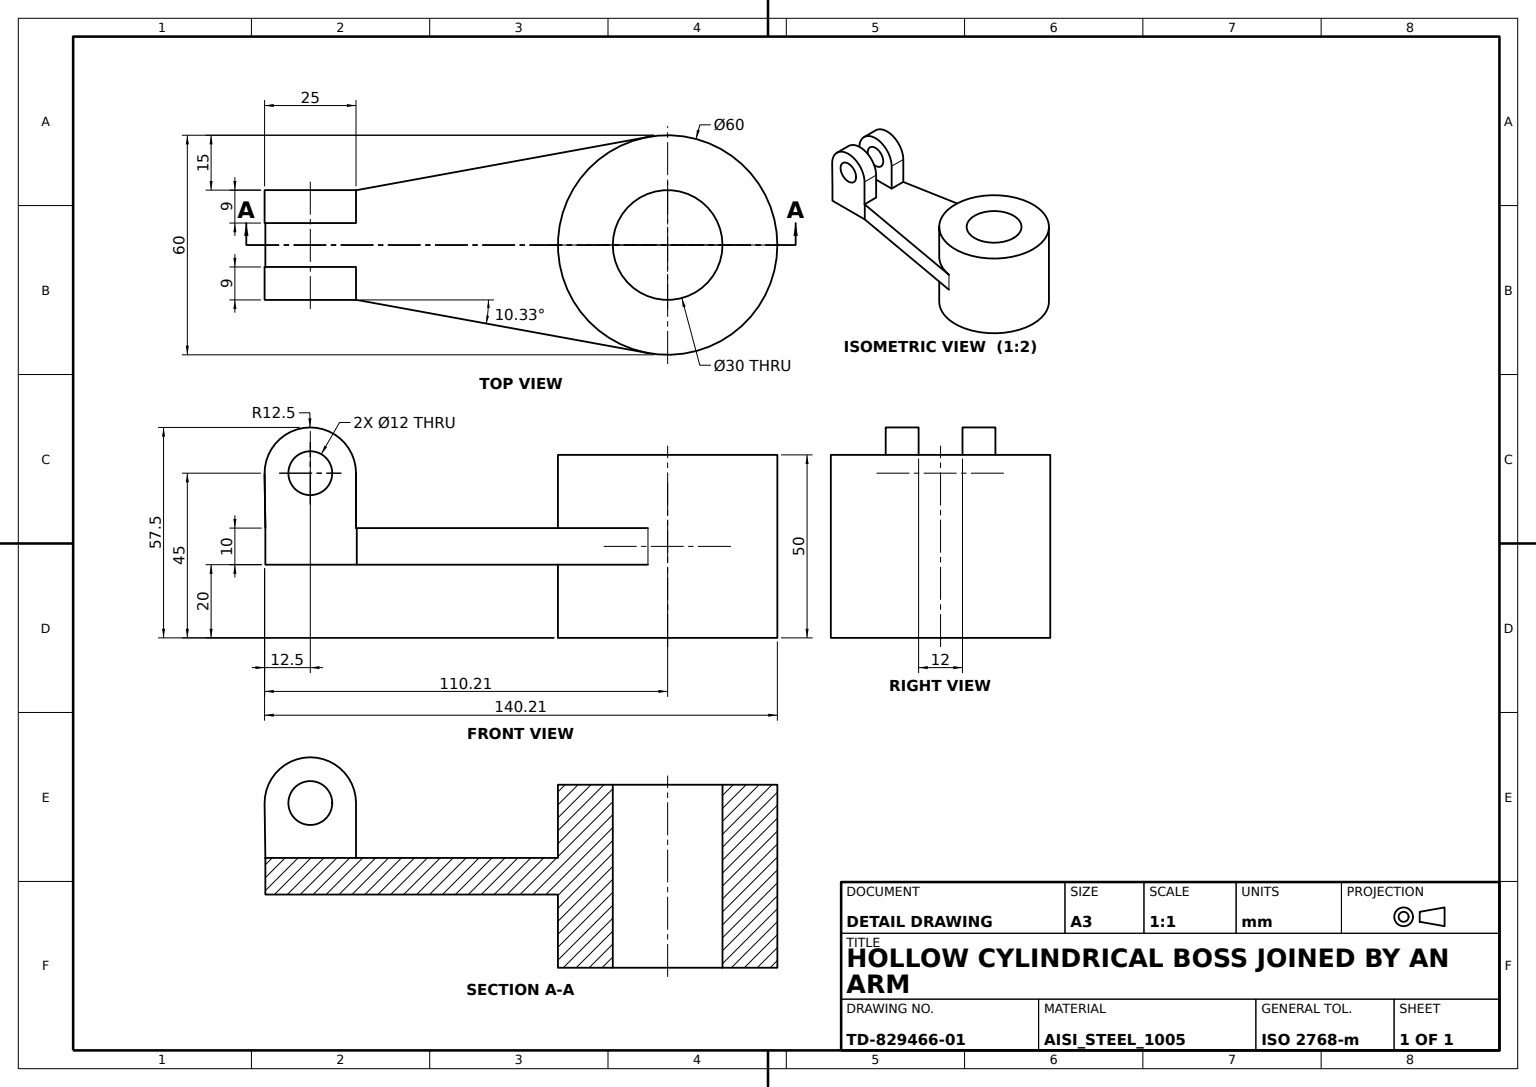
ISO-10303-21;
HEADER;
FILE_DESCRIPTION((''),'2;1');
FILE_NAME('','',(''),(''),'','','');
FILE_SCHEMA(('AUTOMOTIVE_DESIGN'));
ENDSEC;
DATA;
#1=APPLICATION_CONTEXT('');
#2=PRODUCT_CONTEXT('',#1,'mechanical');
#3=PRODUCT('','','',(#2));
#4=PRODUCT_DEFINITION_FORMATION('','',#3);
#5=PRODUCT_DEFINITION_CONTEXT('',#1,'design');
#6=PRODUCT_DEFINITION('','',#4,#5);
#7=PRODUCT_DEFINITION_SHAPE('','',#6);
#8=(LENGTH_UNIT()NAMED_UNIT(*)SI_UNIT(.MILLI.,.METRE.));
#9=(NAMED_UNIT(*)PLANE_ANGLE_UNIT()SI_UNIT($,.RADIAN.));
#10=(NAMED_UNIT(*)SI_UNIT($,.STERADIAN.)SOLID_ANGLE_UNIT());
#11=UNCERTAINTY_MEASURE_WITH_UNIT(LENGTH_MEASURE(0.005),#8,'distance_accuracy_value','');
#12=(GEOMETRIC_REPRESENTATION_CONTEXT(3)GLOBAL_UNCERTAINTY_ASSIGNED_CONTEXT((#11))GLOBAL_UNIT_ASSIGNED_CONTEXT((#8,#9,#10))REPRESENTATION_CONTEXT('',''));
#13=CARTESIAN_POINT('',(-85.210715,-6.,20.));
#14=VERTEX_POINT('',#13);
#15=CARTESIAN_POINT('',(-85.210715,-6.,5.));
#16=VERTEX_POINT('',#15);
#17=DIRECTION('',(0.,0.,-1.));
#18=VECTOR('',#17,1000.);
#19=LINE('',#13,#18);
#20=EDGE_CURVE('',#14,#16,#19,.T.);
#21=ORIENTED_EDGE('',*,*,#20,.F.);
#22=CARTESIAN_POINT('',(-85.210715,-15.,20.));
#23=VERTEX_POINT('',#22);
#24=DIRECTION('',(0.,-1.,0.));
#25=VECTOR('',#24,1000.);
#26=LINE('',#13,#25);
#27=EDGE_CURVE('',#14,#23,#26,.T.);
#28=ORIENTED_EDGE('',*,*,#27,.T.);
#29=CARTESIAN_POINT('',(-85.210715,-15.,5.));
#30=VERTEX_POINT('',#29);
#31=LINE('',#22,#18);
#32=EDGE_CURVE('',#23,#30,#31,.T.);
#33=ORIENTED_EDGE('',*,*,#32,.T.);
#34=LINE('',#15,#25);
#35=EDGE_CURVE('',#16,#30,#34,.T.);
#36=ORIENTED_EDGE('',*,*,#35,.F.);
#37=EDGE_LOOP('',(#21,#28,#33,#36));
#38=FACE_BOUND('',#37,.T.);
#39=DIRECTION('',(-1.,0.,0.));
#40=DIRECTION('',(0.,0.,1.));
#41=AXIS2_PLACEMENT_3D('',#13,#39,#40);
#42=PLANE('',#41);
#43=ADVANCED_FACE('',(#38),#42,.F.);
#44=CARTESIAN_POINT('',(-85.,15.,5.));
#45=VERTEX_POINT('',#44);
#46=CARTESIAN_POINT('',(-85.210715,15.,5.));
#47=VERTEX_POINT('',#46);
#48=VECTOR('',#39,1000.);
#49=LINE('',#44,#48);
#50=EDGE_CURVE('',#45,#47,#49,.T.);
#51=ORIENTED_EDGE('',*,*,#50,.T.);
#52=CARTESIAN_POINT('',(-85.210715,6.,5.));
#53=VERTEX_POINT('',#52);
#54=DIRECTION('',(0.,1.,0.));
#55=VECTOR('',#54,1000.);
#56=LINE('',#52,#55);
#57=EDGE_CURVE('',#53,#47,#56,.T.);
#58=ORIENTED_EDGE('',*,*,#57,.F.);
#59=CARTESIAN_POINT('',(-110.,6.,5.));
#60=VERTEX_POINT('',#59);
#61=LINE('',#52,#48);
#62=EDGE_CURVE('',#53,#60,#61,.T.);
#63=ORIENTED_EDGE('',*,*,#62,.T.);
#64=CARTESIAN_POINT('',(-110.,-6.,5.));
#65=VERTEX_POINT('',#64);
#66=CARTESIAN_POINT('',(-110.,15.,5.));
#67=LINE('',#66,#25);
#68=EDGE_CURVE('',#60,#65,#67,.T.);
#69=ORIENTED_EDGE('',*,*,#68,.T.);
#70=LINE('',#15,#48);
#71=EDGE_CURVE('',#16,#65,#70,.T.);
#72=ORIENTED_EDGE('',*,*,#71,.F.);
#73=ORIENTED_EDGE('',*,*,#35,.T.);
#74=CARTESIAN_POINT('',(-85.,-15.,5.));
#75=VERTEX_POINT('',#74);
#76=CARTESIAN_POINT('',(-110.,-15.,5.));
#77=DIRECTION('',(1.,0.,0.));
#78=VECTOR('',#77,1000.);
#79=LINE('',#76,#78);
#80=EDGE_CURVE('',#30,#75,#79,.T.);
#81=ORIENTED_EDGE('',*,*,#80,.T.);
#82=CARTESIAN_POINT('',(-5.379942,-29.513662,5.));
#83=VERTEX_POINT('',#82);
#84=DIRECTION('',(0.983788721,-0.179331402,0.));
#85=VECTOR('',#84,1000.);
#86=LINE('',#74,#85);
#87=EDGE_CURVE('',#75,#83,#86,.T.);
#88=ORIENTED_EDGE('',*,*,#87,.T.);
#89=CARTESIAN_POINT('',(-5.379942,29.513662,5.));
#90=VERTEX_POINT('',#89);
#91=CARTESIAN_POINT('',(0.,0.,5.));
#92=AXIS2_PLACEMENT_3D('',#91,#17,#77);
#93=CIRCLE('',#92,30.);
#94=EDGE_CURVE('',#83,#90,#93,.T.);
#95=ORIENTED_EDGE('',*,*,#94,.T.);
#96=DIRECTION('',(-0.983788721,-0.179331402,0.));
#97=VECTOR('',#96,1000.);
#98=LINE('',#89,#97);
#99=EDGE_CURVE('',#90,#45,#98,.T.);
#100=ORIENTED_EDGE('',*,*,#99,.T.);
#101=EDGE_LOOP('',(#51,#58,#63,#69,#72,#73,#81,#88,#95,#100));
#102=FACE_BOUND('',#101,.T.);
#103=AXIS2_PLACEMENT_3D('',#91,#17,#39);
#104=PLANE('',#103);
#105=ADVANCED_FACE('',(#102),#104,.F.);
#106=CARTESIAN_POINT('',(-110.209467,-6.,19.823382));
#107=VERTEX_POINT('',#106);
#108=DIRECTION('',(-0.014129422,0.,0.999900175));
#109=VECTOR('',#108,1000.);
#110=LINE('',#64,#109);
#111=EDGE_CURVE('',#65,#107,#110,.T.);
#112=ORIENTED_EDGE('',*,*,#111,.F.);
#113=VERTEX_POINT('',#76);
#114=LINE('',#64,#25);
#115=EDGE_CURVE('',#65,#113,#114,.T.);
#116=ORIENTED_EDGE('',*,*,#115,.T.);
#117=CARTESIAN_POINT('',(-110.209467,-15.,19.823382));
#118=VERTEX_POINT('',#117);
#119=LINE('',#76,#109);
#120=EDGE_CURVE('',#113,#118,#119,.T.);
#121=ORIENTED_EDGE('',*,*,#120,.T.);
#122=LINE('',#106,#25);
#123=EDGE_CURVE('',#107,#118,#122,.T.);
#124=ORIENTED_EDGE('',*,*,#123,.F.);
#125=EDGE_LOOP('',(#112,#116,#121,#124));
#126=FACE_BOUND('',#125,.T.);
#127=DIRECTION('',(0.999900175,0.,0.014129422));
#128=DIRECTION('',(0.014129422,0.,-0.999900175));
#129=AXIS2_PLACEMENT_3D('',#64,#127,#128);
#130=PLANE('',#129);
#131=ADVANCED_FACE('',(#126),#130,.F.);
#132=CARTESIAN_POINT('',(15.,0.,25.));
#133=VERTEX_POINT('',#132);
#134=CARTESIAN_POINT('',(0.,0.,25.));
#135=AXIS2_PLACEMENT_3D('',#134,#40,#77);
#136=CIRCLE('',#135,15.);
#137=EDGE_CURVE('',#133,#133,#136,.T.);
#138=ORIENTED_EDGE('',*,*,#137,.T.);
#139=EDGE_LOOP('',(#138));
#140=FACE_BOUND('',#139,.T.);
#141=CARTESIAN_POINT('',(15.,0.,-25.));
#142=VERTEX_POINT('',#141);
#143=CARTESIAN_POINT('',(0.,0.,-25.));
#144=AXIS2_PLACEMENT_3D('',#143,#40,#77);
#145=CIRCLE('',#144,15.);
#146=EDGE_CURVE('',#142,#142,#145,.T.);
#147=ORIENTED_EDGE('',*,*,#146,.F.);
#148=EDGE_LOOP('',(#147));
#149=FACE_BOUND('',#148,.T.);
#150=AXIS2_PLACEMENT_3D('',#134,#17,#39);
#151=CYLINDRICAL_SURFACE('',#150,15.);
#152=ADVANCED_FACE('',(#140,#149),#151,.F.);
#153=VERTEX_POINT('',#66);
#154=CARTESIAN_POINT('',(-110.,15.,-5.));
#155=VERTEX_POINT('',#154);
#156=LINE('',#66,#18);
#157=EDGE_CURVE('',#153,#155,#156,.T.);
#158=ORIENTED_EDGE('',*,*,#157,.T.);
#159=CARTESIAN_POINT('',(-110.,-15.,-5.));
#160=VERTEX_POINT('',#159);
#161=LINE('',#154,#25);
#162=EDGE_CURVE('',#155,#160,#161,.T.);
#163=ORIENTED_EDGE('',*,*,#162,.T.);
#164=LINE('',#76,#18);
#165=EDGE_CURVE('',#113,#160,#164,.T.);
#166=ORIENTED_EDGE('',*,*,#165,.F.);
#167=ORIENTED_EDGE('',*,*,#115,.F.);
#168=ORIENTED_EDGE('',*,*,#68,.F.);
#169=EDGE_CURVE('',#153,#60,#67,.T.);
#170=ORIENTED_EDGE('',*,*,#169,.F.);
#171=EDGE_LOOP('',(#158,#163,#166,#167,#168,#170));
#172=FACE_BOUND('',#171,.T.);
#173=AXIS2_PLACEMENT_3D('',#66,#77,#17);
#174=PLANE('',#173);
#175=ADVANCED_FACE('',(#172),#174,.F.);
#176=CARTESIAN_POINT('',(-110.209467,6.,19.823382));
#177=VERTEX_POINT('',#176);
#178=CARTESIAN_POINT('',(-85.210715,6.,20.));
#179=VERTEX_POINT('',#178);
#180=CARTESIAN_POINT('',(-97.710715,6.,20.));
#181=AXIS2_PLACEMENT_3D('',#180,#54,#77);
#182=CIRCLE('',#181,12.5);
#183=EDGE_CURVE('',#177,#179,#182,.T.);
#184=ORIENTED_EDGE('',*,*,#183,.T.);
#185=CARTESIAN_POINT('',(-85.210715,15.,20.));
#186=VERTEX_POINT('',#185);
#187=LINE('',#178,#55);
#188=EDGE_CURVE('',#179,#186,#187,.T.);
#189=ORIENTED_EDGE('',*,*,#188,.T.);
#190=CARTESIAN_POINT('',(-110.209467,15.,19.823382));
#191=VERTEX_POINT('',#190);
#192=CARTESIAN_POINT('',(-97.710715,15.,20.));
#193=AXIS2_PLACEMENT_3D('',#192,#54,#77);
#194=CIRCLE('',#193,12.5);
#195=EDGE_CURVE('',#191,#186,#194,.T.);
#196=ORIENTED_EDGE('',*,*,#195,.F.);
#197=LINE('',#176,#55);
#198=EDGE_CURVE('',#177,#191,#197,.T.);
#199=ORIENTED_EDGE('',*,*,#198,.F.);
#200=EDGE_LOOP('',(#184,#189,#196,#199));
#201=FACE_BOUND('',#200,.T.);
#202=AXIS2_PLACEMENT_3D('',#180,#54,#40);
#203=CYLINDRICAL_SURFACE('',#202,12.5);
#204=ADVANCED_FACE('',(#201),#203,.T.);
#205=CARTESIAN_POINT('',(30.,0.,-25.));
#206=VERTEX_POINT('',#205);
#207=CIRCLE('',#144,30.);
#208=EDGE_CURVE('',#206,#206,#207,.T.);
#209=ORIENTED_EDGE('',*,*,#208,.F.);
#210=EDGE_LOOP('',(#209));
#211=FACE_BOUND('',#210,.T.);
#212=ORIENTED_EDGE('',*,*,#146,.T.);
#213=EDGE_LOOP('',(#212));
#214=FACE_BOUND('',#213,.T.);
#215=PLANE('',#144);
#216=ADVANCED_FACE('',(#211,#214),#215,.F.);
#217=CARTESIAN_POINT('',(-91.710715,6.,20.));
#218=VERTEX_POINT('',#217);
#219=AXIS2_PLACEMENT_3D('',#180,#24,#77);
#220=CIRCLE('',#219,6.);
#221=EDGE_CURVE('',#218,#218,#220,.T.);
#222=ORIENTED_EDGE('',*,*,#221,.T.);
#223=EDGE_LOOP('',(#222));
#224=FACE_BOUND('',#223,.T.);
#225=CARTESIAN_POINT('',(-91.710715,15.,20.));
#226=VERTEX_POINT('',#225);
#227=AXIS2_PLACEMENT_3D('',#192,#24,#77);
#228=CIRCLE('',#227,6.);
#229=EDGE_CURVE('',#226,#226,#228,.T.);
#230=ORIENTED_EDGE('',*,*,#229,.F.);
#231=EDGE_LOOP('',(#230));
#232=FACE_BOUND('',#231,.T.);
#233=CYLINDRICAL_SURFACE('',#202,6.);
#234=ADVANCED_FACE('',(#224,#232),#233,.F.);
#235=CARTESIAN_POINT('',(-97.710715,-15.,20.));
#236=AXIS2_PLACEMENT_3D('',#235,#54,#77);
#237=CIRCLE('',#236,12.5);
#238=EDGE_CURVE('',#118,#23,#237,.T.);
#239=ORIENTED_EDGE('',*,*,#238,.F.);
#240=ORIENTED_EDGE('',*,*,#120,.F.);
#241=ORIENTED_EDGE('',*,*,#165,.T.);
#242=CARTESIAN_POINT('',(-85.,-15.,-5.));
#243=VERTEX_POINT('',#242);
#244=LINE('',#159,#78);
#245=EDGE_CURVE('',#160,#243,#244,.T.);
#246=ORIENTED_EDGE('',*,*,#245,.T.);
#247=LINE('',#74,#18);
#248=EDGE_CURVE('',#75,#243,#247,.T.);
#249=ORIENTED_EDGE('',*,*,#248,.F.);
#250=ORIENTED_EDGE('',*,*,#80,.F.);
#251=ORIENTED_EDGE('',*,*,#32,.F.);
#252=EDGE_LOOP('',(#239,#240,#241,#246,#249,#250,#251));
#253=FACE_BOUND('',#252,.T.);
#254=CARTESIAN_POINT('',(-91.710715,-15.,20.));
#255=VERTEX_POINT('',#254);
#256=AXIS2_PLACEMENT_3D('',#235,#24,#77);
#257=CIRCLE('',#256,6.);
#258=EDGE_CURVE('',#255,#255,#257,.T.);
#259=ORIENTED_EDGE('',*,*,#258,.F.);
#260=EDGE_LOOP('',(#259));
#261=FACE_BOUND('',#260,.T.);
#262=AXIS2_PLACEMENT_3D('',#76,#54,#39);
#263=PLANE('',#262);
#264=ADVANCED_FACE('',(#253,#261),#263,.F.);
#265=ORIENTED_EDGE('',*,*,#238,.T.);
#266=ORIENTED_EDGE('',*,*,#27,.F.);
#267=CARTESIAN_POINT('',(-97.710715,-6.,20.));
#268=AXIS2_PLACEMENT_3D('',#267,#54,#77);
#269=CIRCLE('',#268,12.5);
#270=EDGE_CURVE('',#107,#14,#269,.T.);
#271=ORIENTED_EDGE('',*,*,#270,.F.);
#272=ORIENTED_EDGE('',*,*,#123,.T.);
#273=EDGE_LOOP('',(#265,#266,#271,#272));
#274=FACE_BOUND('',#273,.T.);
#275=AXIS2_PLACEMENT_3D('',#267,#24,#17);
#276=CYLINDRICAL_SURFACE('',#275,12.5);
#277=ADVANCED_FACE('',(#274),#276,.T.);
#278=ORIENTED_EDGE('',*,*,#137,.F.);
#279=EDGE_LOOP('',(#278));
#280=FACE_BOUND('',#279,.T.);
#281=CARTESIAN_POINT('',(30.,0.,25.));
#282=VERTEX_POINT('',#281);
#283=CIRCLE('',#135,30.);
#284=EDGE_CURVE('',#282,#282,#283,.T.);
#285=ORIENTED_EDGE('',*,*,#284,.T.);
#286=EDGE_LOOP('',(#285));
#287=FACE_BOUND('',#286,.T.);
#288=PLANE('',#135);
#289=ADVANCED_FACE('',(#280,#287),#288,.T.);
#290=CARTESIAN_POINT('',(-85.,15.,-5.));
#291=VERTEX_POINT('',#290);
#292=LINE('',#44,#18);
#293=EDGE_CURVE('',#45,#291,#292,.T.);
#294=ORIENTED_EDGE('',*,*,#293,.F.);
#295=ORIENTED_EDGE('',*,*,#99,.F.);
#296=CARTESIAN_POINT('',(-5.379942,29.513662,-5.));
#297=VERTEX_POINT('',#296);
#298=LINE('',#89,#18);
#299=EDGE_CURVE('',#90,#297,#298,.T.);
#300=ORIENTED_EDGE('',*,*,#299,.T.);
#301=LINE('',#296,#97);
#302=EDGE_CURVE('',#297,#291,#301,.T.);
#303=ORIENTED_EDGE('',*,*,#302,.T.);
#304=EDGE_LOOP('',(#294,#295,#300,#303));
#305=FACE_BOUND('',#304,.T.);
#306=DIRECTION('',(0.179331402,-0.983788721,0.));
#307=DIRECTION('',(0.983788721,0.179331402,0.));
#308=AXIS2_PLACEMENT_3D('',#89,#306,#307);
#309=PLANE('',#308);
#310=ADVANCED_FACE('',(#305),#309,.F.);
#311=ORIENTED_EDGE('',*,*,#258,.T.);
#312=EDGE_LOOP('',(#311));
#313=FACE_BOUND('',#312,.T.);
#314=CARTESIAN_POINT('',(-91.710715,-6.,20.));
#315=VERTEX_POINT('',#314);
#316=AXIS2_PLACEMENT_3D('',#267,#24,#77);
#317=CIRCLE('',#316,6.);
#318=EDGE_CURVE('',#315,#315,#317,.T.);
#319=ORIENTED_EDGE('',*,*,#318,.F.);
#320=EDGE_LOOP('',(#319));
#321=FACE_BOUND('',#320,.T.);
#322=CYLINDRICAL_SURFACE('',#275,6.);
#323=ADVANCED_FACE('',(#313,#321),#322,.F.);
#324=ORIENTED_EDGE('',*,*,#169,.T.);
#325=LINE('',#59,#109);
#326=EDGE_CURVE('',#60,#177,#325,.T.);
#327=ORIENTED_EDGE('',*,*,#326,.T.);
#328=ORIENTED_EDGE('',*,*,#198,.T.);
#329=LINE('',#66,#109);
#330=EDGE_CURVE('',#153,#191,#329,.T.);
#331=ORIENTED_EDGE('',*,*,#330,.F.);
#332=EDGE_LOOP('',(#324,#327,#328,#331));
#333=FACE_BOUND('',#332,.T.);
#334=DIRECTION('',(-0.999900175,0.,-0.014129422));
#335=AXIS2_PLACEMENT_3D('',#59,#334,#108);
#336=PLANE('',#335);
#337=ADVANCED_FACE('',(#333),#336,.T.);
#338=ORIENTED_EDGE('',*,*,#299,.F.);
#339=ORIENTED_EDGE('',*,*,#94,.F.);
#340=CARTESIAN_POINT('',(-5.379942,-29.513662,-5.));
#341=VERTEX_POINT('',#340);
#342=LINE('',#82,#18);
#343=EDGE_CURVE('',#83,#341,#342,.T.);
#344=ORIENTED_EDGE('',*,*,#343,.T.);
#345=CARTESIAN_POINT('',(0.,0.,-5.));
#346=AXIS2_PLACEMENT_3D('',#345,#17,#77);
#347=CIRCLE('',#346,30.);
#348=EDGE_CURVE('',#341,#297,#347,.T.);
#349=ORIENTED_EDGE('',*,*,#348,.T.);
#350=EDGE_LOOP('',(#338,#339,#344,#349));
#351=FACE_BOUND('',#350,.T.);
#352=ORIENTED_EDGE('',*,*,#284,.F.);
#353=EDGE_LOOP('',(#352));
#354=FACE_BOUND('',#353,.T.);
#355=ORIENTED_EDGE('',*,*,#208,.T.);
#356=EDGE_LOOP('',(#355));
#357=FACE_BOUND('',#356,.T.);
#358=CYLINDRICAL_SURFACE('',#150,30.);
#359=ADVANCED_FACE('',(#351,#354,#357),#358,.T.);
#360=ORIENTED_EDGE('',*,*,#318,.T.);
#361=EDGE_LOOP('',(#360));
#362=FACE_BOUND('',#361,.T.);
#363=ORIENTED_EDGE('',*,*,#20,.T.);
#364=ORIENTED_EDGE('',*,*,#71,.T.);
#365=ORIENTED_EDGE('',*,*,#111,.T.);
#366=ORIENTED_EDGE('',*,*,#270,.T.);
#367=EDGE_LOOP('',(#363,#364,#365,#366));
#368=FACE_BOUND('',#367,.T.);
#369=AXIS2_PLACEMENT_3D('',#267,#54,#40);
#370=PLANE('',#369);
#371=ADVANCED_FACE('',(#362,#368),#370,.T.);
#372=ORIENTED_EDGE('',*,*,#248,.T.);
#373=LINE('',#242,#85);
#374=EDGE_CURVE('',#243,#341,#373,.T.);
#375=ORIENTED_EDGE('',*,*,#374,.T.);
#376=ORIENTED_EDGE('',*,*,#343,.F.);
#377=ORIENTED_EDGE('',*,*,#87,.F.);
#378=EDGE_LOOP('',(#372,#375,#376,#377));
#379=FACE_BOUND('',#378,.T.);
#380=DIRECTION('',(0.179331402,0.983788721,0.));
#381=DIRECTION('',(-0.983788721,0.179331402,0.));
#382=AXIS2_PLACEMENT_3D('',#74,#380,#381);
#383=PLANE('',#382);
#384=ADVANCED_FACE('',(#379),#383,.F.);
#385=ORIENTED_EDGE('',*,*,#162,.F.);
#386=LINE('',#290,#48);
#387=EDGE_CURVE('',#291,#155,#386,.T.);
#388=ORIENTED_EDGE('',*,*,#387,.F.);
#389=ORIENTED_EDGE('',*,*,#302,.F.);
#390=ORIENTED_EDGE('',*,*,#348,.F.);
#391=ORIENTED_EDGE('',*,*,#374,.F.);
#392=ORIENTED_EDGE('',*,*,#245,.F.);
#393=EDGE_LOOP('',(#385,#388,#389,#390,#391,#392));
#394=FACE_BOUND('',#393,.T.);
#395=AXIS2_PLACEMENT_3D('',#345,#17,#39);
#396=PLANE('',#395);
#397=ADVANCED_FACE('',(#394),#396,.T.);
#398=ORIENTED_EDGE('',*,*,#195,.T.);
#399=LINE('',#185,#18);
#400=EDGE_CURVE('',#186,#47,#399,.T.);
#401=ORIENTED_EDGE('',*,*,#400,.T.);
#402=ORIENTED_EDGE('',*,*,#50,.F.);
#403=ORIENTED_EDGE('',*,*,#293,.T.);
#404=ORIENTED_EDGE('',*,*,#387,.T.);
#405=ORIENTED_EDGE('',*,*,#157,.F.);
#406=ORIENTED_EDGE('',*,*,#330,.T.);
#407=EDGE_LOOP('',(#398,#401,#402,#403,#404,#405,#406));
#408=FACE_BOUND('',#407,.T.);
#409=ORIENTED_EDGE('',*,*,#229,.T.);
#410=EDGE_LOOP('',(#409));
#411=FACE_BOUND('',#410,.T.);
#412=AXIS2_PLACEMENT_3D('',#44,#24,#77);
#413=PLANE('',#412);
#414=ADVANCED_FACE('',(#408,#411),#413,.F.);
#415=ORIENTED_EDGE('',*,*,#57,.T.);
#416=ORIENTED_EDGE('',*,*,#400,.F.);
#417=ORIENTED_EDGE('',*,*,#188,.F.);
#418=LINE('',#178,#18);
#419=EDGE_CURVE('',#179,#53,#418,.T.);
#420=ORIENTED_EDGE('',*,*,#419,.T.);
#421=EDGE_LOOP('',(#415,#416,#417,#420));
#422=FACE_BOUND('',#421,.T.);
#423=AXIS2_PLACEMENT_3D('',#178,#77,#17);
#424=PLANE('',#423);
#425=ADVANCED_FACE('',(#422),#424,.T.);
#426=ORIENTED_EDGE('',*,*,#221,.F.);
#427=EDGE_LOOP('',(#426));
#428=FACE_BOUND('',#427,.T.);
#429=ORIENTED_EDGE('',*,*,#326,.F.);
#430=ORIENTED_EDGE('',*,*,#62,.F.);
#431=ORIENTED_EDGE('',*,*,#419,.F.);
#432=ORIENTED_EDGE('',*,*,#183,.F.);
#433=EDGE_LOOP('',(#429,#430,#431,#432));
#434=FACE_BOUND('',#433,.T.);
#435=PLANE('',#202);
#436=ADVANCED_FACE('',(#428,#434),#435,.F.);
#437=CLOSED_SHELL('',(#43,#105,#131,#152,#175,#204,#216,#234,#264,#277,#289,#310,#323,#337,#359,#371,#384,#397,#414,#425,#436));
#438=MANIFOLD_SOLID_BREP('',#437);
#439=ADVANCED_BREP_SHAPE_REPRESENTATION('',(#438),#12);
#440=SHAPE_DEFINITION_REPRESENTATION(#7,#439);
ENDSEC;
END-ISO-10303-21;
